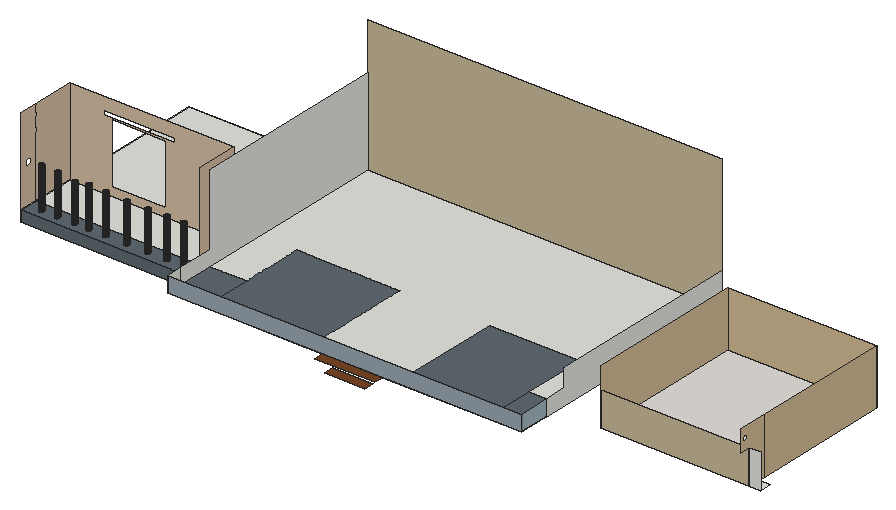
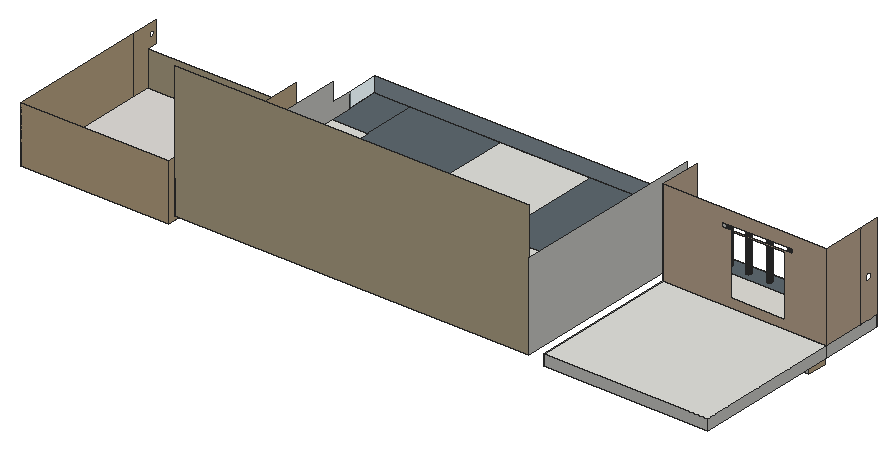
# SketchUp Ruby script. Lengths in inches.
U = 1.inch
M = Sketchup.active_model
def pt(a) = Geom::Point3d.new(a.map { |v| v * U })
def face(e, loops, mat)
  f = e.add_face(loops[0].map { |a| pt(a) })
  loops[1..].each { |l| e.add_face(l.map { |a| pt(a) }).erase! }
  f.material = f.back_material = mat if mat
  f
end
# faces: each face lists its corners as indices into pts; further lists are holes
def faces(e, pts, list, mat = nil) = list.each { |f| face(e, (f[0].is_a?(Array) ? f : [f]).map { |l| l.map { |i| pts[i] } }, mat) }
# xy, xz, yz: faces in a plane at the given z, y or x. An outline is a flat list of corners, or four numbers for a rectangle; further outlines are holes
def ring(l) = l.size == 4 ? [[l[0], l[1]], [l[2], l[1]], [l[2], l[3]], [l[0], l[3]]] : l.each_slice(2).to_a
def flat(e, list, mat, &to3) = list.each { |f| face(e, (f[0].is_a?(Array) ? f : [f]).map { |l| ring(l).map { |u, v| to3.(u, v) } }, mat) }
def xy(e, z, list, mat = nil) = flat(e, list, mat) { |x, y| [x, y, z] }
def xz(e, y, list, mat = nil) = flat(e, list, mat) { |x, z| [x, y, z] }
def yz(e, x, list, mat = nil) = flat(e, list, mat) { |y, z| [x, y, z] }
def lines(e, pts, list) = list.each { |a, b| e.add_line(pt(pts[a]), pt(pts[b])) }
# prism: a flat outline (further loops are holes) pulled along v
def prism(e, loops, v, mat = nil)
  f = face(e, loops, mat); d = Geom::Vector3d.new(v.map { |x| x * U })
  f.pushpull(f.normal.samedirection?(d) ? d.length : -d.length)
end
def box(e, o, s, mat = nil) = prism(e, [[o, [o[0] + s[0], o[1], o[2]], [o[0] + s[0], o[1] + s[1], o[2]], [o[0], o[1] + s[1], o[2]]]], [0, 0, s[2]], mat)
def at(x, y, z, deg = 0) = Geom::Transformation.translation(pt([x, y, z])) * Geom::Transformation.rotation(ORIGIN, Z_AXIS, deg.degrees)
def axes(o, x, y, z) = Geom::Transformation.new([*x, 0, *y, 0, *z, 0, *pt(o).to_a, 1])
def part(name) = M.definitions.add(name)
# library, detail: a bought-in or finely detailed component or shape, given as its bounding box
def library(name, o, s) = part(name).tap { |d| box(d.entities, o, s) }
def detail(e, o, s) = box(e.add_group.entities, o, s)
def put(e, d, t, mat = nil) = e.add_instance(d, t).tap { |i| i.material = mat if mat }
def group(e, t, mat = nil) = e.add_group.tap { |g| g.transformation = t; g.material = mat if mat }.entities
root = M.entities
M.materials.add("[Formica Beige]").color = [211, 187, 149]
M.materials.add("[Formica Laminate Dark]").color = [50, 53, 60]
M.materials.add("[Formica Laminate Light]").color = [213, 189, 164]
M.materials.add("[Formica Speckled Grey]").color = [94, 105, 111]
M.materials.add("[Marble Carrara Gold Floor Tile]").color = [225, 223, 217]
M.materials.add("[Quartz Light Brown]").color = [199, 184, 152]
M.materials.add("[Terrazzo Light Blue]").color = [151, 165, 175]
M.materials.add("[Terrazzo Tile Accent]").color = [224, 221, 217]
M.materials.add("[Translucent Glass Safety]").color = [204, 235, 244]
M.materials["[Translucent Glass Safety]"].alpha = 0.5
M.materials.add("[Wood Veneer 01]2").color = [120, 70, 37]
xy(root,609.74,[[28.72,169.65,143.97,191.15]],"[Formica Beige]")
xy(root,617.3,[[28.72,169.65,143.97,191.15]],"[Formica Beige]")
xy(root,621,[[774.15,169.39,786.87,182.57]])
xy(root,621,[[611.125,169.39,774.15,344.36]],"[Terrazzo Tile Accent]")
xy(root,633,[[9,191.15,189.57,355.125]])
xy(root,633,[[9,122.79,189.57,191.15]],"[Formica Beige]")
xy(root,634.57,[[380.3,77.26,424.94,88.2]],"[Wood Veneer 01]2")
xy(root,645,[[351.88,88.2,351.88,216.84,238.58,216.84,238.58,147.05,198.57,147.05,198.57,364.125,588.3,364.125,588.3,147.05,549.2,147.05,549.2,216.84,450.54,216.84,450.54,88.2],[23.62,130.88,22.9375,130.97,22.3,131.23,21.76,131.65,21.34,132.19,21.08,132.82,20.99,133.5,21.08,134.18,21.34,134.81,21.76,135.36,22.3,135.78,22.9375,136.04,23.62,136.13,24.29,136.04,24.93,135.78,25.47,135.36,25.89,134.81,26.15,134.18,26.24,133.5,26.15,132.82,25.89,132.19,25.47,131.65,24.93,131.23,24.29,130.97],[41.37,130.88,40.6875,130.97,40.05,131.23,39.51,131.65,39.09,132.19,38.83,132.82,38.74,133.5,38.83,134.18,39.09,134.81,39.51,135.36,40.05,135.78,40.6875,136.04,41.37,136.13,42.04,136.04,42.68,135.78,43.22,135.36,43.64,134.81,43.9,134.18,43.99,133.5,43.9,132.82,43.64,132.19,43.22,131.65,42.68,131.23,42.04,130.97],[60.55,130.88,59.875,130.97,59.24,131.23,58.7,131.65,58.28,132.19,58.02,132.82,57.93,133.5,58.02,134.18,58.28,134.81,58.7,135.36,59.24,135.78,59.875,136.04,60.55,136.13,61.23,136.04,61.87,135.78,62.41,135.36,62.83,134.81,63.09,134.18,63.18,133.5,63.09,132.82,62.83,132.19,62.41,131.65,61.87,131.23,61.23,130.97],[75.99,130.88,75.3125,130.97,74.68,131.23,74.13,131.65,73.72,132.19,73.45,132.82,73.37,133.5,73.45,134.18,73.72,134.81,74.13,135.36,74.68,135.78,75.3125,136.04,75.99,136.13,76.67,136.04,77.3,135.78,77.85,135.36,78.26,134.81,78.53,134.18,78.62,133.5,78.53,132.82,78.26,132.19,77.85,131.65,77.3,131.23,76.67,130.97],
  [94.37,130.88,93.6875,130.97,93.05,131.23,92.51,131.65,92.09,132.19,91.83,132.82,91.74,133.5,91.83,134.18,92.09,134.81,92.51,135.36,93.05,135.78,93.6875,136.04,94.37,136.13,95.04,136.04,95.68,135.78,96.22,135.36,96.64,134.81,96.9,134.18,96.99,133.5,96.9,132.82,96.64,132.19,96.22,131.65,95.68,131.23,95.04,130.97],[117.43,130.88,116.75,130.97,116.12,131.23,115.57,131.65,115.15,132.19,114.89,132.82,114.8,133.5,114.89,134.18,115.15,134.81,115.57,135.36,116.12,135.78,116.75,136.04,117.43,136.13,118.11,136.04,118.74,135.78,119.28,135.36,119.7,134.81,119.96,134.18,120.05,133.5,119.96,132.82,119.7,132.19,119.28,131.65,118.74,131.23,118.11,130.97],[140.74,130.88,140.0625,130.97,139.43,131.23,138.88,131.65,138.47,132.19,138.2,132.82,138.12,133.5,138.2,134.18,138.47,134.81,138.88,135.36,139.43,135.78,140.0625,136.04,140.74,136.13,141.42,136.04,142.05,135.78,142.6,135.36,143.01,134.81,143.28,134.18,143.37,133.5,143.28,132.82,143.01,132.19,142.6,131.65,142.05,131.23,141.42,130.97],[161.99,130.88,161.3125,130.97,160.68,131.23,160.13,131.65,159.72,132.19,159.45,132.82,159.37,133.5,159.45,134.18,159.72,134.81,160.13,135.36,160.68,135.78,161.3125,136.04,161.99,136.13,162.67,136.04,163.3,135.78,163.85,135.36,164.26,134.81,164.53,134.18,164.62,133.5,164.53,132.82,164.26,132.19,163.85,131.65,163.3,131.23,162.67,130.97],[179.99,130.88,179.3125,130.97,178.68,131.23,178.13,131.65,177.72,132.19,177.45,132.82,177.37,133.5,177.45,134.18,177.72,134.81,178.13,135.36,178.68,135.78,179.3125,136.04,179.99,136.13,180.67,136.04,181.3,135.78,181.85,135.36,182.26,134.81,182.53,134.18,182.62,133.5,182.53,132.82,182.26,132.19,181.85,131.65,181.3,131.23,180.67,130.97],
  [9,191.15,189.57,355.125]])
xy(root,645,[[198.57,88.2,238.58,147.05],[238.58,88.2,351.88,216.84],[450.54,88.2,549.2,216.84],[549.2,88.2,588.3,147.05],[[9,122.79,189.57,144.21],[179.99,130.88,179.3125,130.97,178.68,131.23,178.13,131.65,177.72,132.19,177.45,132.82,177.37,133.5,177.45,134.18,177.72,134.81,178.13,135.36,178.68,135.78,179.3125,136.04,179.99,136.13,180.67,136.04,181.3,135.78,181.85,135.36,182.26,134.81,182.53,134.18,182.62,133.5,182.53,132.82,182.26,132.19,181.85,131.65,181.3,131.23,180.67,130.97],[41.37,130.88,40.6875,130.97,40.05,131.23,39.51,131.65,39.09,132.19,38.83,132.82,38.74,133.5,38.83,134.18,39.09,134.81,39.51,135.36,40.05,135.78,40.6875,136.04,41.37,136.13,42.04,136.04,42.68,135.78,43.22,135.36,43.64,134.81,43.9,134.18,43.99,133.5,43.9,132.82,43.64,132.19,43.22,131.65,42.68,131.23,42.04,130.97],[161.99,130.88,161.3125,130.97,160.68,131.23,160.13,131.65,159.72,132.19,159.45,132.82,159.37,133.5,159.45,134.18,159.72,134.81,160.13,135.36,160.68,135.78,161.3125,136.04,161.99,136.13,162.67,136.04,163.3,135.78,163.85,135.36,164.26,134.81,164.53,134.18,164.62,133.5,164.53,132.82,164.26,132.19,163.85,131.65,163.3,131.23,162.67,130.97],[60.55,130.88,59.875,130.97,59.24,131.23,58.7,131.65,58.28,132.19,58.02,132.82,57.93,133.5,58.02,134.18,58.28,134.81,58.7,135.36,59.24,135.78,59.875,136.04,60.55,136.13,61.23,136.04,61.87,135.78,62.41,135.36,62.83,134.81,63.09,134.18,63.18,133.5,63.09,132.82,62.83,132.19,62.41,131.65,61.87,131.23,61.23,130.97],[140.74,130.88,140.0625,130.97,139.43,131.23,138.88,131.65,138.47,132.19,138.2,132.82,138.12,133.5,138.2,134.18,138.47,134.81,138.88,135.36,139.43,135.78,140.0625,136.04,140.74,136.13,141.42,136.04,142.05,135.78,142.6,135.36,143.01,134.81,143.28,134.18,143.37,133.5,143.28,132.82,143.01,132.19,142.6,131.65,142.05,131.23,141.42,130.97],[75.99,130.88,75.3125,130.97,74.68,131.23,74.13,131.65,73.72,132.19,73.45,132.82,73.37,133.5,73.45,134.18,73.72,134.81,74.13,135.36,74.68,135.78,75.3125,136.04,75.99,136.13,76.67,136.04,77.3,135.78,77.85,135.36,78.26,134.81,78.53,134.18,78.62,133.5,78.53,132.82,78.26,132.19,77.85,131.65,77.3,131.23,76.67,130.97],[117.43,130.88,116.75,130.97,116.12,131.23,115.57,131.65,115.15,132.19,114.89,132.82,114.8,133.5,114.89,134.18,115.15,134.81,115.57,135.36,116.12,135.78,116.75,136.04,117.43,136.13,118.11,136.04,118.74,135.78,119.28,135.36,119.7,134.81,119.96,134.18,120.05,133.5,119.96,132.82,119.7,132.19,119.28,131.65,118.74,131.23,118.11,130.97],[94.37,130.88,93.6875,130.97,93.05,131.23,92.51,131.65,92.09,132.19,91.83,132.82,91.74,133.5,91.83,134.18,92.09,134.81,92.51,135.36,93.05,135.78,93.6875,136.04,94.37,136.13,95.04,136.04,95.68,135.78,96.22,135.36,96.64,134.81,96.9,134.18,96.99,133.5,96.9,132.82,96.64,132.19,96.22,131.65,95.68,131.23,95.04,130.97],[23.62,130.88,22.9375,130.97,22.3,131.23,21.76,131.65,21.34,132.19,21.08,132.82,20.99,133.5,21.08,134.18,21.34,134.81,21.76,135.36,22.3,135.78,22.9375,136.04,23.62,136.13,24.29,136.04,24.93,135.78,25.47,135.36,25.89,134.81,26.15,134.18,26.24,133.5,26.15,132.82,25.89,132.19,25.47,131.65,24.93,131.23,24.29,130.97]]],"[Formica Speckled Grey]")
xy(root,645,[[9,144.21,189.57,191.15]],"[Marble Carrara Gold Floor Tile]")
xy(root,645,[[369.87,77.26,435.37,88.2]],"[Wood Veneer 01]2")
xz(root,88.2,[[198.57,645,588.3,662.0625]],"[Terrazzo Light Blue]")
xz(root,122.79,[[9,633,189.57,645]],"[Formica Speckled Grey]")
xz(root,169.39,[[774.15,621,786.87,658.875]])
xz(root,169.39,[[611.125,621,774.15,658.875]],"[Quartz Light Brown]")
xz(root,169.65,[[28.72,609.74,143.97,617.3]],"[Formica Beige]")
xz(root,191.15,[[28.72,609.74,143.97,617.3]])
xz(root,191.15,[[[9,645,189.57,740.5625],[54.875,654.41,114.625,720.78],[46.64,721.83,124.14,726.77]]],"[Formica Laminate Light]")
xz(root,344.36,[[611.125,621,774.15,682.5]],"[Formica Beige]")
xz(root,355.125,[[9,633,189.57,645]])
xz(root,364.125,[[198.57,645,588.3,793.1875]],"[Quartz Light Brown]")
yz(root,9,[[122.79,633,191.15,645],[191.15,633,355.125,645]])
yz(root,9,[[[122.79,645,144.21,740.5625],[133.5,683.96,132.53,684.08,131.63,684.46,130.85,685.06,130.25,685.83,129.88,686.74,129.75,687.71,129.88,688.68,130.25,689.58,130.85,690.36,131.63,690.95,132.53,691.33,133.5,691.46,134.47,691.33,135.38,690.95,136.15,690.36,136.75,689.58,137.125,688.68,137.25,687.71,137.125,686.74,136.75,685.83,136.15,685.06,135.38,684.46,134.47,684.08]],[144.21,645,191.15,740.5625]],"[Formica Laminate Light]")
yz(root,28.72,[[169.65,609.74,191.15,617.3]],"[Formica Beige]")
yz(root,143.97,[[169.65,609.74,191.15,617.3]],"[Formica Beige]")
yz(root,189.57,[[122.79,633,191.15,645],[191.15,633,355.125,645]])
yz(root,189.57,[[144.21,645,191.15,740.5625]],"[Formica Laminate Light]")
yz(root,198.57,[[88.2,645,105.54,662.0625],[105.54,645,364.125,645,364.125,740.5625,147.05,740.5625,147.05,662.0625,105.54,662.0625]])
yz(root,588.3,[[122.79,645,122.79,662.0625,147.05,662.0625,147.05,682.5,364.125,682.5,364.125,645]])
yz(root,588.3,[[88.2,645,122.79,662.0625]],"[Translucent Glass Safety]")
yz(root,611.125,[[169.39,621,344.36,682.5]],"[Formica Beige]")
yz(root,774.15,[[[169.39,621,169.39,658.875,157.7,658.875,157.7,682.5,189.24,682.5,189.24,621],[163.52,668.49,164.28,668.59,164.99,668.89,165.6,669.35,166.07,669.96,166.36,670.67,166.46,671.43,166.36,672.19,166.07,672.9,165.6,673.51,164.99,673.97,164.28,674.27,163.52,674.37,162.76,674.27,162.06,673.97,161.45,673.51,160.98,672.9,160.6875,672.19,160.59,671.43,160.6875,670.67,160.98,669.96,161.45,669.35,162.06,668.89,162.76,668.59]],[189.24,621,344.36,682.5]],"[Formica Beige]")
p = [[22.9375,130.97,645],[23.62,130.88,645],[23.62,130.88,690.36],[22.9375,130.97,690.36],[24.29,130.97,645],[24.29,130.97,690.36],
  [40.6875,130.97,645],[41.37,130.88,645],[41.37,130.88,689.58],[40.6875,130.97,689.58],[42.04,130.97,645],[42.04,130.97,689.58],
  [59.875,130.97,645],[60.55,130.88,645],[60.55,130.88,686.625],[59.875,130.97,686.625],[61.23,130.97,645],[61.23,130.97,686.625],
  [75.3125,130.97,645],[75.99,130.88,645],[75.99,130.88,689.58],[75.3125,130.97,689.58],[76.67,130.97,645],[76.67,130.97,689.58],
  [93.6875,130.97,645],[94.37,130.88,645],[94.37,130.88,688.6875],[93.6875,130.97,688.6875],[95.04,130.97,645],[95.04,130.97,688.6875],
  [116.75,130.97,645],[117.43,130.88,645],[117.43,130.88,687.6875],[116.75,130.97,687.6875],[118.11,130.97,645],[118.11,130.97,687.6875],
  [140.0625,130.97,645],[140.74,130.88,645],[140.74,130.88,688.0625],[140.0625,130.97,688.0625],[141.42,130.97,645],[141.42,130.97,688.0625],
  [161.3125,130.97,645],[161.99,130.88,645],[161.99,130.88,688.68],[161.3125,130.97,688.68],[162.67,130.97,645],[162.67,130.97,688.68],
  [179.3125,130.97,645],[179.99,130.88,645],[179.99,130.88,688.5],[179.3125,130.97,688.5],[180.67,130.97,645],[180.67,130.97,688.5],
  [22.3,131.23,645],[22.3,131.23,690.36],[24.93,131.23,645],[24.93,131.23,690.36],[40.05,131.23,645],[40.05,131.23,689.58],
  [42.68,131.23,645],[42.68,131.23,689.58],[59.24,131.23,645],[59.24,131.23,686.625],[61.87,131.23,645],[61.87,131.23,686.625],
  [74.68,131.23,645],[74.68,131.23,689.58],[77.3,131.23,645],[77.3,131.23,689.58],[93.05,131.23,645],[93.05,131.23,688.6875],
  [95.68,131.23,645],[95.68,131.23,688.6875],[116.12,131.23,645],[116.12,131.23,687.6875],[118.74,131.23,645],[118.74,131.23,687.6875],
  [139.43,131.23,645],[139.43,131.23,688.0625],[142.05,131.23,645],[142.05,131.23,688.0625],[160.68,131.23,645],[160.68,131.23,688.68],
  [163.3,131.23,645],[163.3,131.23,688.68],[178.68,131.23,645],[178.68,131.23,688.5],[181.3,131.23,645],[181.3,131.23,688.5],
  [21.76,131.65,645],[21.76,131.65,690.36],[25.47,131.65,645],[25.47,131.65,690.36],[39.51,131.65,645],[39.51,131.65,689.58],
  [43.22,131.65,645],[43.22,131.65,689.58],[58.7,131.65,645],[58.7,131.65,686.625],[62.41,131.65,645],[62.41,131.65,686.625],
  [74.13,131.65,645],[74.13,131.65,689.58],[77.85,131.65,645],[77.85,131.65,689.58],[92.51,131.65,645],[92.51,131.65,688.6875],
  [96.22,131.65,645],[96.22,131.65,688.6875],[115.57,131.65,645],[115.57,131.65,687.6875],[119.28,131.65,645],[119.28,131.65,687.6875],
  [138.88,131.65,645],[138.88,131.65,688.0625],[142.6,131.65,645],[142.6,131.65,688.0625],[160.13,131.65,645],[160.13,131.65,688.68],
  [163.85,131.65,645],[163.85,131.65,688.68],[178.13,131.65,645],[178.13,131.65,688.5],[181.85,131.65,645],[181.85,131.65,688.5],
  [21.34,132.19,645],[21.34,132.19,690.36],[25.89,132.19,645],[25.89,132.19,690.36],[39.09,132.19,645],[39.09,132.19,689.58],
  [43.64,132.19,645],[43.64,132.19,689.58],[58.28,132.19,645],[58.28,132.19,686.625],[62.83,132.19,645],[62.83,132.19,686.625],
  [73.72,132.19,645],[73.72,132.19,689.58],[78.26,132.19,645],[78.26,132.19,689.58],[92.09,132.19,645],[92.09,132.19,688.6875],
  [96.64,132.19,645],[96.64,132.19,688.6875],[115.15,132.19,645],[115.15,132.19,687.6875],[119.7,132.19,645],[119.7,132.19,687.6875],
  [138.47,132.19,645],[138.47,132.19,688.0625],[143.01,132.19,645],[143.01,132.19,688.0625],[159.72,132.19,645],[159.72,132.19,688.68],
  [164.26,132.19,645],[164.26,132.19,688.68],[177.72,132.19,645],[177.72,132.19,688.5],[182.26,132.19,645],[182.26,132.19,688.5],
  [21.08,132.82,645],[21.08,132.82,690.36],[26.15,132.82,645],[26.15,132.82,690.36],[38.83,132.82,645],[38.83,132.82,689.58],
  [43.9,132.82,645],[43.9,132.82,689.58],[58.02,132.82,645],[58.02,132.82,686.625],[63.09,132.82,645],[63.09,132.82,686.625],
  [73.45,132.82,645],[73.45,132.82,689.58],[78.53,132.82,645],[78.53,132.82,689.58],[91.83,132.82,645],[91.83,132.82,688.6875],
  [96.9,132.82,645],[96.9,132.82,688.6875],[114.89,132.82,645],[114.89,132.82,687.6875],[119.96,132.82,645],[119.96,132.82,687.6875],
  [138.2,132.82,645],[138.2,132.82,688.0625],[143.28,132.82,645],[143.28,132.82,688.0625],[159.45,132.82,645],[159.45,132.82,688.68],
  [164.53,132.82,645],[164.53,132.82,688.68],[177.45,132.82,645],[177.45,132.82,688.5],[182.53,132.82,645],[182.53,132.82,688.5],
  [20.99,133.5,645],[20.99,133.5,690.36],[20.99,133.5,683.96],[26.24,133.5,645],[26.24,133.5,683.96],[26.24,133.5,690.36],
  [38.74,133.5,645],[38.74,133.5,689.58],[38.74,133.5,683.96],[43.99,133.5,645],[43.99,133.5,683.96],[43.99,133.5,689.58],
  [57.93,133.5,645],[57.93,133.5,686.625],[57.93,133.5,683.96],[63.18,133.5,645],[63.18,133.5,683.96],[63.18,133.5,686.625],
  [73.37,133.5,645],[73.37,133.5,689.58],[73.37,133.5,683.96],[78.62,133.5,645],[78.62,133.5,683.96],[78.62,133.5,689.58],
  [91.74,133.5,645],[91.74,133.5,688.6875],[91.74,133.5,683.96],[96.99,133.5,645],[96.99,133.5,683.96],[96.99,133.5,688.6875],
  [114.8,133.5,645],[114.8,133.5,687.6875],[114.8,133.5,683.96],[120.05,133.5,645],[120.05,133.5,683.96],[120.05,133.5,687.6875],
  [138.12,133.5,645],[138.12,133.5,688.0625],[138.12,133.5,683.96],[143.37,133.5,645],[143.37,133.5,683.96],[143.37,133.5,688.0625],
  [159.37,133.5,645],[159.37,133.5,688.68],[159.37,133.5,683.96],[164.62,133.5,645],[164.62,133.5,683.96],[164.62,133.5,688.68],
  [177.37,133.5,645],[177.37,133.5,688.5],[177.37,133.5,683.96],[182.62,133.5,645],[182.62,133.5,683.96],[182.62,133.5,688.5],
  [21.08,134.18,645],[21.08,134.18,690.36],[26.15,134.18,645],[26.15,134.18,690.36],[38.83,134.18,645],[38.83,134.18,689.58],
  [43.9,134.18,645],[43.9,134.18,689.58],[58.02,134.18,645],[58.02,134.18,686.625],[63.09,134.18,645],[63.09,134.18,686.625],
  [73.45,134.18,645],[73.45,134.18,689.58],[78.53,134.18,645],[78.53,134.18,689.58],[91.83,134.18,645],[91.83,134.18,688.6875],
  [96.9,134.18,645],[96.9,134.18,688.6875],[114.89,134.18,645],[114.89,134.18,687.6875],[119.96,134.18,645],[119.96,134.18,687.6875],
  [138.2,134.18,645],[138.2,134.18,688.0625],[143.28,134.18,645],[143.28,134.18,688.0625],[159.45,134.18,645],[159.45,134.18,688.68],
  [164.53,134.18,645],[164.53,134.18,688.68],[177.45,134.18,645],[177.45,134.18,688.5],[182.53,134.18,645],[182.53,134.18,688.5],
  [21.34,134.81,645],[21.34,134.81,690.36],[25.89,134.81,645],[25.89,134.81,690.36],[39.09,134.81,645],[39.09,134.81,689.58],
  [43.64,134.81,645],[43.64,134.81,689.58],[58.28,134.81,645],[58.28,134.81,686.625],[62.83,134.81,645],[62.83,134.81,686.625],
  [73.72,134.81,645],[73.72,134.81,689.58],[78.26,134.81,645],[78.26,134.81,689.58],[92.09,134.81,645],[92.09,134.81,688.6875],
  [96.64,134.81,645],[96.64,134.81,688.6875],[115.15,134.81,645],[115.15,134.81,687.6875],[119.7,134.81,645],[119.7,134.81,687.6875],
  [138.47,134.81,645],[138.47,134.81,688.0625],[143.01,134.81,645],[143.01,134.81,688.0625],[159.72,134.81,645],[159.72,134.81,688.68],
  [164.26,134.81,645],[164.26,134.81,688.68],[177.72,134.81,645],[177.72,134.81,688.5],[182.26,134.81,645],[182.26,134.81,688.5],
  [21.76,135.36,645],[21.76,135.36,690.36],[25.47,135.36,645],[25.47,135.36,690.36],[39.51,135.36,645],[39.51,135.36,689.58],
  [43.22,135.36,645],[43.22,135.36,689.58],[58.7,135.36,645],[58.7,135.36,686.625],[62.41,135.36,645],[62.41,135.36,686.625],
  [74.13,135.36,645],[74.13,135.36,689.58],[77.85,135.36,645],[77.85,135.36,689.58],[92.51,135.36,645],[92.51,135.36,688.6875],
  [96.22,135.36,645],[96.22,135.36,688.6875],[115.57,135.36,645],[115.57,135.36,687.6875],[119.28,135.36,645],[119.28,135.36,687.6875],
  [138.88,135.36,645],[138.88,135.36,688.0625],[142.6,135.36,645],[142.6,135.36,688.0625],[160.13,135.36,645],[160.13,135.36,688.68],
  [163.85,135.36,645],[163.85,135.36,688.68],[178.13,135.36,645],[178.13,135.36,688.5],[181.85,135.36,645],[181.85,135.36,688.5],
  [22.3,135.78,645],[22.3,135.78,690.36],[24.93,135.78,645],[24.93,135.78,690.36],[40.05,135.78,645],[40.05,135.78,689.58],
  [42.68,135.78,645],[42.68,135.78,689.58],[59.24,135.78,645],[59.24,135.78,686.625],[61.87,135.78,645],[61.87,135.78,686.625],
  [74.68,135.78,645],[74.68,135.78,689.58],[77.3,135.78,645],[77.3,135.78,689.58],[93.05,135.78,645],[93.05,135.78,688.6875],
  [95.68,135.78,645],[95.68,135.78,688.6875],[116.12,135.78,645],[116.12,135.78,687.6875],[118.74,135.78,645],[118.74,135.78,687.6875],
  [139.43,135.78,645],[139.43,135.78,688.0625],[142.05,135.78,645],[142.05,135.78,688.0625],[160.68,135.78,645],[160.68,135.78,688.68],
  [163.3,135.78,645],[163.3,135.78,688.68],[178.68,135.78,645],[178.68,135.78,688.5],[181.3,135.78,645],[181.3,135.78,688.5],
  [22.9375,136.04,645],[22.9375,136.04,690.36],[24.29,136.04,645],[24.29,136.04,690.36],[40.6875,136.04,645],[40.6875,136.04,689.58],
  [42.04,136.04,645],[42.04,136.04,689.58],[59.875,136.04,645],[59.875,136.04,686.625],[61.23,136.04,645],[61.23,136.04,686.625],
  [75.3125,136.04,645],[75.3125,136.04,689.58],[76.67,136.04,645],[76.67,136.04,689.58],[93.6875,136.04,645],[93.6875,136.04,688.6875],
  [95.04,136.04,645],[95.04,136.04,688.6875],[116.75,136.04,645],[116.75,136.04,687.6875],[118.11,136.04,645],[118.11,136.04,687.6875],
  [140.0625,136.04,645],[140.0625,136.04,688.0625],[141.42,136.04,645],[141.42,136.04,688.0625],[161.3125,136.04,645],[161.3125,136.04,688.68],
  [162.67,136.04,645],[162.67,136.04,688.68],[179.3125,136.04,645],[179.3125,136.04,688.5],[180.67,136.04,645],[180.67,136.04,688.5],
  [23.62,136.13,645],[23.62,136.13,690.36],[41.37,136.13,645],[41.37,136.13,689.58],[60.55,136.13,645],[60.55,136.13,686.625],
  [75.99,136.13,645],[75.99,136.13,689.58],[94.37,136.13,645],[94.37,136.13,688.6875],[117.43,136.13,645],[117.43,136.13,687.6875],
  [140.74,136.13,645],[140.74,136.13,688.0625],[161.99,136.13,645],[161.99,136.13,688.68],[179.99,136.13,645],[179.99,136.13,688.5]]
faces(root,p,[[0,1,2,3],[1,4,5,2],[6,7,8,9],[7,10,11,8],[12,13,14,15],[13,16,17,14],[18,19,20,21],[19,22,23,20],
  [24,25,26,27],[25,28,29,26],[30,31,32,33],[31,34,35,32],[36,37,38,39],[37,40,41,38],[42,43,44,45],[43,46,47,44],
  [48,49,50,51],[49,52,53,50],[54,0,3,55],[4,56,57,5],[58,6,9,59],[10,60,61,11],[62,12,15,63],[16,64,65,17],
  [66,18,21,67],[22,68,69,23],[70,24,27,71],[28,72,73,29],[74,30,33,75],[34,76,77,35],[78,36,39,79],[40,80,81,41],
  [82,42,45,83],[46,84,85,47],[86,48,51,87],[52,88,89,53],[90,54,55,91],[56,92,93,57],[94,58,59,95],[60,96,97,61],
  [98,62,63,99],[64,100,101,65],[102,66,67,103],[68,104,105,69],[106,70,71,107],[72,108,109,73],[110,74,75,111],[76,112,113,77],
  [114,78,79,115],[80,116,117,81],[118,82,83,119],[84,120,121,85],[122,86,87,123],[88,124,125,89],[126,90,91,127],[92,128,129,93],
  [130,94,95,131],[96,132,133,97],[134,98,99,135],[100,136,137,101],[138,102,103,139],[104,140,141,105],[142,106,107,143],[108,144,145,109],
  [146,110,111,147],[112,148,149,113],[150,114,115,151],[116,152,153,117],[154,118,119,155],[120,156,157,121],[158,122,123,159],[124,160,161,125],
  [162,126,127,163],[128,164,165,129],[166,130,131,167],[132,168,169,133],[170,134,135,171],[136,172,173,137],[174,138,139,175],[140,176,177,141],
  [178,142,143,179],[144,180,181,145],[182,146,147,183],[148,184,185,149],[186,150,151,187],[152,188,189,153],[190,154,155,191],[156,192,193,157],
  [194,158,159,195],[160,196,197,161],[198,162,163,199,200],[164,201,202,203,165],[204,166,167,205,206],[168,207,208,209,169],[210,170,171,211,212],[172,213,214,215,173],
  [216,174,175,217,218],[176,219,220,221,177],[222,178,179,223,224],[180,225,226,227,181],[228,182,183,229,230],[184,231,232,233,185],[234,186,187,235,236],[188,237,238,239,189],
  [240,190,191,241,242],[192,243,244,245,193],[246,194,195,247,248],[196,249,250,251,197],[252,198,200,199,253],[201,254,255,203,202],[256,204,206,205,257],[207,258,259,209,208],
  [260,210,212,211,261],[213,262,263,215,214],[264,216,218,217,265],[219,266,267,221,220],[268,222,224,223,269],[225,270,271,227,226],[272,228,230,229,273],[231,274,275,233,232],
  [276,234,236,235,277],[237,278,279,239,238],[280,240,242,241,281],[243,282,283,245,244],[284,246,248,247,285],[249,286,287,251,250],[288,252,253,289],[254,290,291,255],
  [292,256,257,293],[258,294,295,259],[296,260,261,297],[262,298,299,263],[300,264,265,301],[266,302,303,267],[304,268,269,305],[270,306,307,271],
  [308,272,273,309],[274,310,311,275],[312,276,277,313],[278,314,315,279],[316,280,281,317],[282,318,319,283],[320,284,285,321],[286,322,323,287],
  [324,288,289,325],[290,326,327,291],[328,292,293,329],[294,330,331,295],[332,296,297,333],[298,334,335,299],[336,300,301,337],[302,338,339,303],
  [340,304,305,341],[306,342,343,307],[344,308,309,345],[310,346,347,311],[348,312,313,349],[314,350,351,315],[352,316,317,353],[318,354,355,319],
  [356,320,321,357],[322,358,359,323],[360,324,325,361],[326,362,363,327],[364,328,329,365],[330,366,367,331],[368,332,333,369],[334,370,371,335],
  [372,336,337,373],[338,374,375,339],[376,340,341,377],[342,378,379,343],[380,344,345,381],[346,382,383,347],[384,348,349,385],[350,386,387,351],
  [388,352,353,389],[354,390,391,355],[392,356,357,393],[358,394,395,359],[396,360,361,397],[362,398,399,363],[400,364,365,401],[366,402,403,367],
  [404,368,369,405],[370,406,407,371],[408,372,373,409],[374,410,411,375],[412,376,377,413],[378,414,415,379],[416,380,381,417],[382,418,419,383],
  [420,384,385,421],[386,422,423,387],[424,388,389,425],[390,426,427,391],[428,392,393,429],[394,430,431,395],[432,396,397,433],[398,432,433,399],
  [434,400,401,435],[402,434,435,403],[436,404,405,437],[406,436,437,407],[438,408,409,439],[410,438,439,411],[440,412,413,441],[414,440,441,415],
  [442,416,417,443],[418,442,443,419],[444,420,421,445],[422,444,445,423],[446,424,425,447],[426,446,447,427],[448,428,429,449],[430,448,449,431]],"[Formica Laminate Dark]")
